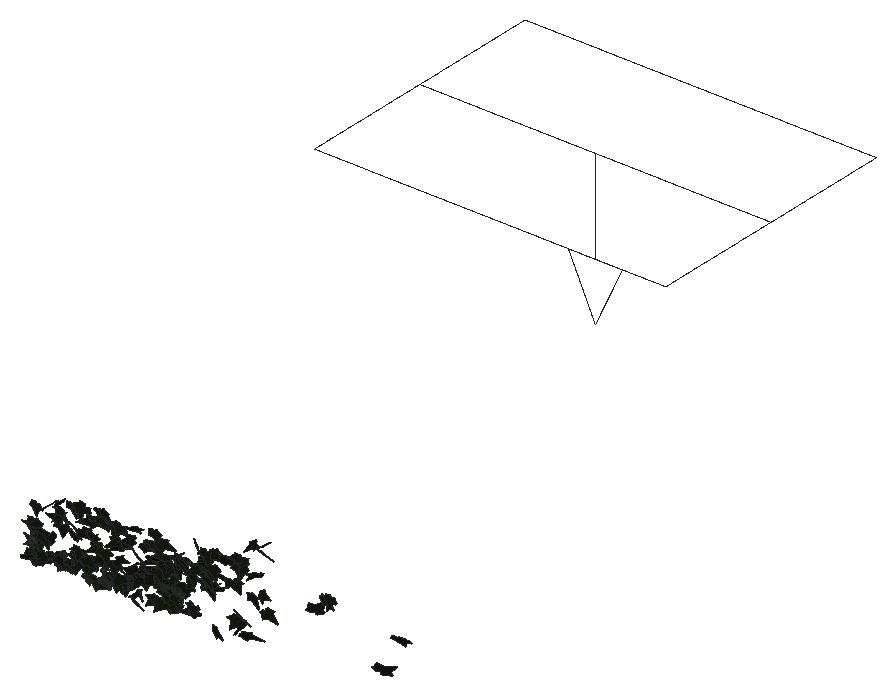
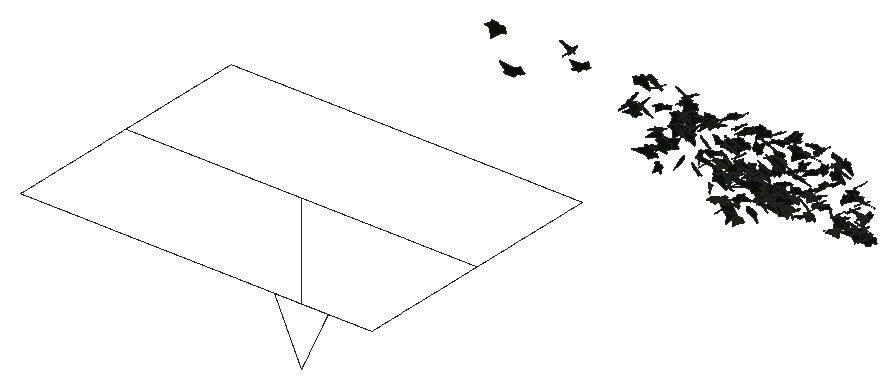
# SketchUp Ruby script. Lengths in millimetres.
U = 1.mm
M = Sketchup.active_model
def pt(a) = Geom::Point3d.new(a.map { |v| v * U })
def face(e, loops, mat)
  f = e.add_face(loops[0].map { |a| pt(a) })
  loops[1..].each { |l| e.add_face(l.map { |a| pt(a) }).erase! }
  f.material = f.back_material = mat if mat
  f
end
# faces: each face lists its corners as indices into pts; further lists are holes
def faces(e, pts, list, mat = nil) = list.each { |f| face(e, (f[0].is_a?(Array) ? f : [f]).map { |l| l.map { |i| pts[i] } }, mat) }
# xy, xz, yz: faces in a plane at the given z, y or x. An outline is a flat list of corners, or four numbers for a rectangle; further outlines are holes
def ring(l) = l.size == 4 ? [[l[0], l[1]], [l[2], l[1]], [l[2], l[3]], [l[0], l[3]]] : l.each_slice(2).to_a
def flat(e, list, mat, &to3) = list.each { |f| face(e, (f[0].is_a?(Array) ? f : [f]).map { |l| ring(l).map { |u, v| to3.(u, v) } }, mat) }
def xy(e, z, list, mat = nil) = flat(e, list, mat) { |x, y| [x, y, z] }
def xz(e, y, list, mat = nil) = flat(e, list, mat) { |x, z| [x, y, z] }
def yz(e, x, list, mat = nil) = flat(e, list, mat) { |y, z| [x, y, z] }
def lines(e, pts, list) = list.each { |a, b| e.add_line(pt(pts[a]), pt(pts[b])) }
# prism: a flat outline (further loops are holes) pulled along v
def prism(e, loops, v, mat = nil)
  f = face(e, loops, mat); d = Geom::Vector3d.new(v.map { |x| x * U })
  f.pushpull(f.normal.samedirection?(d) ? d.length : -d.length)
end
def box(e, o, s, mat = nil) = prism(e, [[o, [o[0] + s[0], o[1], o[2]], [o[0] + s[0], o[1] + s[1], o[2]], [o[0], o[1] + s[1], o[2]]]], [0, 0, s[2]], mat)
def at(x, y, z, deg = 0) = Geom::Transformation.translation(pt([x, y, z])) * Geom::Transformation.rotation(ORIGIN, Z_AXIS, deg.degrees)
def axes(o, x, y, z) = Geom::Transformation.new([*x, 0, *y, 0, *z, 0, *pt(o).to_a, 1])
def part(name) = M.definitions.add(name)
# library, detail: a bought-in or finely detailed component or shape, given as its bounding box
def library(name, o, s) = part(name).tap { |d| box(d.entities, o, s) }
def detail(e, o, s) = box(e.add_group.entities, o, s)
def put(e, d, t, mat = nil) = e.add_instance(d, t).tap { |i| i.material = mat if mat }
def group(e, t, mat = nil) = e.add_group.tap { |g| g.transformation = t; g.material = mat if mat }.entities
root = M.entities
M.materials.add("efeu1").color = [18, 25, 13]
M.materials.add("efeu2").color = [43, 57, 29]
c1 = part("ivyleaf_9")
p = [[39.1,54.8,31.7],[34.5,51.8,30.2],[-5.3,25.2,17.3],[-17.9,28.3,20.9],[-21.6,21.7,17],[-20.2,4.3,5.3],
  [-22.9,-0.3,2.5],[-17.1,-4,-0.6],[-2,-2.1,-1.2],[-0.7,-15.4,-10.1],[16.6,-22.3,-16.7],[21.1,-15.1,-12.5],
  [32.7,-10.7,-11],[46.1,-1.8,-6.6],[30.8,11.2,3.8]]
faces(c1.entities,p,[[0,1,2,3,4,5,6,7,8,9,10,11,12,13,14]],"efeu1")
c2 = part("ivyleaf_10")
p = [[0,12.8,-0.8],[-1.5,51.3,-10.9],[-4.9,51,-11.6],[-13.6,26.5,-7.3],[-13.2,15.9,-4.6],[-21.1,19.3,-7.2],
  [-29.5,16.3,-8.3],[-29.2,8.3,-6.2],[-19.7,-9.8,0.5],[-7.6,-13,4],[1,-12.2,5.8],[-0.4,51.1,-11.1],
  [-1.5,51.1,-10.9],[1,-12.4,5.9],[16.9,-12.4,3.5],[35.1,9.1,-5.1],[35,12.9,-6.1],[20.5,16.4,-4.9],
  [15.8,15,-3.8],[15.3,27.6,-7.1],[12.8,31.3,-7.8]]
faces(c2.entities,p,[[0,1,2,3,4,5,6,7,8,9,10],[11,12,0,13,14,15,16,17,18,19,20]],"efeu2")
c3 = part("Group257\#1")
p = [[0,0,0],[0,0,-959.4],[-272.7,0,-959.4],[1775.1,-1330.8,0],[-1775.1,-1330.8,0],[1775.1,1330.8,0],
  [1775.1,0,0],[-1775.1,1330.8,0],[272.7,0,-959.4],[-1775.1,0,0],[0,0,-1552.9]]
lines(c3.entities,p,[[0,1],[1,2],[3,4],[5,6],[7,5],[1,8],[9,0],[0,6],[8,10],[4,9],[6,3],[2,10],
  [9,7]])
c4 = part("Rectangle Light\#4")
put(c4.entities,c3,at(0,0,0))
put(root,c1,axes([7078.2,622.4,4794.7],[-1.245,-0.97894,0.63666],[-0.02381,-0.72384,-1.12583],[2.22236,-0.55617,0.34461]))
put(root,c2,axes([6934.9,593.1,4256.7],[-2.21181,-0.09357,-0.49205],[0.94502,-0.0521,-1.16284],[0.12508,-1.26095,0.08456]))
put(root,c1,axes([6281,585,4503.6],[2.52907,0.12258,-0.03253],[-0.06178,-0.00223,-1.33449],[-0.23333,1.32925,0.00076]))
put(root,c1,axes([6495.9,585.8,4670.1],[-1.29976,0.62888,0.92752],[-1.25598,0.65217,-0.92809],[-1.72371,-0.94941,-0.02314]))
put(root,c1,axes([6590.3,616.6,4820.6],[0.27311,-1.35729,0.14133],[0.01392,-0.14134,-1.36483],[2.59711,0.14349,-0.00755]))
put(root,c1,axes([6466.9,608.1,4738.9],[0.97787,-1.23155,-0.18048],[-0.14465,0.16385,-1.33441],[2.3645,0.51934,-0.00699]))
put(root,c1,axes([6744.1,595.8,4396.6],[0.64791,-0.91908,-0.92115],[-0.18486,0.93155,-0.96535],[2.46961,0.31086,0.16941]))
put(root,c1,axes([8009.6,616.5,4759.5],[-0.41068,-1.33295,-0.20263],[0.05642,0.20047,-1.3503],[2.5654,-0.21779,-0.00274]))
put(root,c1,axes([6918.3,615.8,4519.7],[-0.61056,-1.24261,-0.27622],[0.19455,0.25879,-1.28292],[2.41484,-0.33503,0.03352]))
put(root,c1,axes([6622.9,612.8,4311.1],[-1.63327,-0.68293,-0.61293],[0.92945,0.3706,-1.09668],[1.47861,-0.98732,0.01232]))
put(root,c1,axes([8044.7,595.2,4214.7],[1.52551,-0.81377,-0.91631],[-1.19527,0.66743,-1.14212],[2.00281,1.01816,0.01632]))
put(root,c1,axes([7850.7,609.5,4299.7],[-2.33926,0.27794,0.5582],[-1.02866,0.14045,-1.26005],[-0.59186,-1.34261,-0.01626]))
put(root,c1,axes([6390.5,631.9,4433.6],[-0.02071,-0.10759,1.41416],[-1.48401,-1.18083,-0.09584],[2.25466,-0.77821,-0.05009]))
put(root,c1,axes([7276.6,610.4,4576.3],[0.80844,-1.11543,0.79685],[-0.56507,0.73957,1.19352],[-2.54702,-0.51812,-0.01186]))
put(root,c1,axes([6402.3,601.3,4773.2],[-0.77594,1.19359,-0.3546],[0.06299,-0.3626,-1.25859],[-2.36893,-0.4006,0.08268]))
put(root,c1,axes([6634,625.9,4779],[0.47434,-1.23586,0.4161],[0.17935,-0.40546,-1.26069],[2.47534,0.2662,0.01161]))
put(root,c1,axes([7795.2,632,4600.8],[-0.27937,-1.24372,0.49099],[0.16104,-0.50159,-1.24527],[2.53972,-0.10501,0.13297]))
put(root,c1,axes([7504,623.9,4248.5],[-2.12366,-0.60101,-0.02105],[0.03428,0.01095,-1.2674],[1.14403,-1.11598,-0.0011]))
put(root,c1,axes([7229.7,595.6,4449.9],[-1.02657,0.98174,0.63763],[-0.921,0.45227,-1.10571],[-2.02867,-0.70212,0.17932]))
put(root,c1,axes([7208,605.4,4193.2],[2.05762,-0.66884,-0.30097],[-0.37912,0.24818,-1.26709],[1.3434,1.09446,0.1034]))
put(root,c1,axes([7500.5,595.2,4807.4],[0.76205,-0.5492,-1.21421],[0.12929,1.2746,-0.55411],[2.53298,0.10016,0.39358]))
put(root,c1,axes([7266.7,622.8,4393.1],[-2.10613,0.05032,-0.70148],[1.31881,-0.14542,-1.10359],[-0.22867,-1.30213,0.09614]))
put(root,c1,axes([6438.3,617,4296.1],[0.57814,-1.2113,-0.37192],[0.01779,0.38459,-1.24494],[2.41151,0.28756,0.09835]))
put(root,c1,axes([8560.5,606.4,4548.9],[0.61357,-1.05749,-0.93526],[-0.15117,0.94423,-1.09502],[2.68256,0.29508,0.15221]))
put(root,c1,axes([6579,614.5,4643.3],[1.97556,-0.82635,0.11102],[0.19213,-0.05141,-1.32659],[1.57517,1.04268,0.02257]))
put(root,c1,axes([7876.8,631.7,4680.3],[-2.31475,-0.23202,0.40606],[-0.5934,-0.441,-1.18586],[0.6634,-1.20401,0.3561]))
put(root,c1,axes([6132.4,628.2,4373.1],[1.08236,-1.03781,0.44412],[0.51604,-0.35715,-1.1818],[2.08552,0.62698,0.06193]))
put(root,c1,axes([8394.5,626.8,4630.2],[0.75629,-1.31613,-0.09347],[-0.06978,0.08657,-1.37477],[2.51019,0.39894,-0.01006]))
put(root,c1,axes([9717.4,611.8,4417.8],[-0.61084,-0.00029,1.42032],[2.65001,-0.28736,0.31459],[0.53334,1.42749,0.06362]))
put(root,c1,axes([7340.3,602,4731.9],[0.76226,-0.43282,-1.2469],[0.2578,1.30964,-0.41109],[2.49874,-0.00308,0.42279]))
put(root,c1,axes([7437.1,632,4745.2],[-0.19745,-1.33603,-0.1816],[-0.02194,0.18301,-1.33981],[2.56603,-0.10124,-0.02543]))
put(root,c1,axes([6701.1,633.6,4832.6],[-2.38193,-0.47755,-0.07895],[0.14095,0.02737,-1.33955],[0.91035,-1.25373,0.00083]))
put(root,c1,axes([6296.2,631.4,4255],[-2.275,0.08413,-0.39144],[0.70954,-0.21554,-1.18479],[-0.27787,-1.23921,0.1795]))
put(root,c2,axes([6902.4,629.9,4330.1],[1.32405,-1.01667,0.30384],[0.46548,-0.1999,-1.22888],[1.9651,0.73236,0.08637]))
put(root,c1,axes([6823.4,596.4,4598.7],[0.05355,0.16855,-1.30878],[-1.36437,1.101,0.12638],[2.1085,0.70815,0.11502]))
put(root,c1,axes([9893.2,607.7,4777.9],[2.48145,0.60112,-0.31814],[-0.54004,-0.14437,-1.43568],[-1.17637,1.3343,-0.01201]))
put(root,c1,axes([6765.5,631.8,4616.1],[0.9903,-1.19661,-0.04835],[-0.02932,0.04603,-1.30484],[2.27906,0.52054,0.00422]))
put(root,c1,axes([7404.4,636.3,4854.8],[0.27087,-1.32639,-0.08879],[0.03121,0.09104,-1.33375],[2.52984,0.14089,0.02596]))
put(root,c1,axes([7029,603.5,4586.3],[1.66456,0.16047,0.98959],[1.58884,0.61055,-0.83683],[-1.05642,1.1711,0.30068]))
put(root,c1,axes([6243.9,614.6,4501.1],[-1.2524,0.6636,0.93178],[-1.39566,0.5803,-0.93118],[-1.67093,-0.98209,0.07939]))
put(root,c1,axes([6832.8,629.3,4851.8],[1.55402,-1.05267,-0.13594],[-0.10535,0.12904,-1.33177],[2.01733,0.81765,0.03517]))
put(root,c1,axes([6865.1,631.8,4789.6],[0.44276,-1.24833,-0.40414],[0.05236,0.415,-1.26602],[2.49668,0.21267,0.09822]))
put(root,c1,axes([7935.2,642,4853.6],[-0.68157,-1.28837,-0.09768],[0.06076,0.0925,-1.33721],[2.45832,-0.35949,0.00597]))
put(root,c1,axes([8295.1,642,4849.2],[-1.93796,-0.15161,-0.85733],[1.65255,-0.27334,-0.98296],[-0.1212,-1.30275,0.30601]))
put(root,c1,axes([7341.2,626.5,4737.3],[1.50887,-1.05829,-0.35194],[-0.14928,0.37782,-1.31281],[2.11734,0.7808,0.15824]))
put(root,c1,axes([7041.2,643.4,4755.6],[-1.8811,-0.8944,-0.09871],[0.12954,0.0719,-1.33297],[1.70765,-0.9907,-0.00762]))
put(root,c1,axes([6466.8,604.9,4790.9],[-0.05691,1.1823,0.56334],[-0.16238,0.56053,-1.18094],[-2.48724,-0.06365,0.06421]))
put(root,c1,axes([6804.4,634.2,4731.5],[-2.20298,0.25758,0.63395],[-1.22704,0.00692,-1.17999],[-0.43641,-1.31973,0.11755]))
put(root,c1,axes([8260,648.8,4821.3],[-0.6842,-1.26365,0.20168],[0.17219,-0.23406,-1.30528],[2.42932,-0.33931,0.14932]))
put(root,c1,axes([7912.3,629,4586.3],[1.89664,-0.88618,-0.14908],[-0.20508,0.10317,-1.33357],[1.69794,1.00235,0.00546]))
put(root,c1,axes([9184,639.8,4874.8],[-2.14436,0.02339,-0.86278],[1.63757,-0.08103,-1.12584],[-0.12906,-1.41679,0.05015]))
put(root,c1,axes([7055.5,643.2,4323.3],[-2.13545,-0.49957,-0.40756],[0.76754,0.09442,-1.226],[0.95736,-1.19002,0.07382]))
put(root,c1,axes([6884.6,638.7,4854.6],[1.11664,-1.21149,-0.08961],[-0.09766,0.07471,-1.34602],[2.30994,0.5888,-0.01359]))
put(root,c1,axes([7659.6,642.3,4679.4],[0.70748,-1.3592,-0.17061],[-0.05053,0.1696,-1.40899],[2.60664,0.37219,0.01899]))
put(root,c1,axes([8439.3,633.8,4835.9],[0.03758,1.02003,-0.88375],[-0.27518,-0.87716,-1.01566],[-2.55382,0.10952,0.09644]))
put(root,c1,axes([7677.3,644.6,4692.6],[0.85234,-1.22621,0.06593],[0.04279,-0.06198,-1.30544],[2.33671,0.44841,-0.00014]))
put(root,c2,axes([6174.2,628.6,4359.7],[0.82399,1.17989,0.10803],[0.0123,0.11266,-1.25639],[-2.25492,0.43177,0.03262]))
put(root,c1,axes([7397.1,645.7,4413.4],[-2.38769,-0.09063,0.16456],[-0.31226,-0.01264,-1.25783],[0.17414,-1.26525,0.00078]))
put(root,c1,axes([6395.9,644.5,4293.5],[-0.44978,-1.14024,-0.51955],[0.80049,0.42584,-1.12592],[2.2464,-0.38005,0.29719]))
put(root,c1,axes([7189.3,634.2,4701],[-2.12457,0.62863,0.29212],[-0.46369,0.1626,-1.28096],[-1.23511,-1.14239,-0.02158]))
put(root,c1,axes([7775.9,663.1,4293],[-0.62335,-0.97207,0.78046],[-0.41583,-0.74969,-1.02545],[2.33583,-0.39288,0.02572]))
put(root,c1,axes([6107.8,638.5,4168.2],[2.06594,0.69081,0.17384],[-0.28626,-0.08744,1.28666],[1.32517,-1.09586,0.00692]))
put(root,c1,axes([7047.7,614.1,4484.9],[0.30462,0.06924,-1.32906],[-0.62488,1.29931,0.02815],[2.4546,0.32218,0.1721]))
put(root,c1,axes([7711.5,631.5,4703.7],[2.29619,-0.38811,0.45328],[0.9787,0.1575,-1.23388],[0.57619,1.27917,0.28945]))
put(root,c1,axes([8035.3,644.3,4871.9],[-2.25157,0.52033,-0.24498],[0.41055,-0.11794,-1.29225],[-1.01464,-1.20237,0.02074]))
put(root,c1,axes([8230.9,641.2,4409.7],[2.23134,-0.86353,0.02651],[0.0402,-0.01603,-1.4561],[1.64375,1.1726,-0.00038]))
put(root,c1,axes([9107.8,637.2,4855.4],[1.48503,-1.03601,-0.56814],[-0.45325,0.52897,-1.29167],[2.20261,0.80735,0.11725]))
put(root,c1,axes([7657.7,660.7,4691.5],[-1.3952,-1.09231,0.05257],[0.16275,-0.12035,-1.30825],[2.07492,-0.72504,0.13796]))
put(root,c1,axes([6290.2,656.6,4225.1],[-2.09746,-0.62143,0.03852],[-0.05541,-0.02679,-1.26517],[1.18368,-1.10242,0.00903]))
put(root,c1,axes([6466,658.9,4577.3],[-0.78808,-1.25309,-0.00492],[0.04773,-0.00311,-1.3195],[2.38442,-0.4141,0.02479]))
put(root,c1,axes([6453.7,651.2,4672.5],[-0.48978,0.84043,-0.97979],[0.35644,-0.9642,-0.87624],[-2.43077,-0.31073,0.06893]))
put(root,c1,axes([6268.4,654.4,4410.8],[0.03251,-1.28705,-0.21282],[0.03976,0.21308,-1.28695],[2.48246,0.01344,0.0234]))
put(root,c1,axes([6631.9,663.4,4404.1],[-1.07292,-1.14112,0.16814],[-0.08912,-0.16435,-1.27241],[2.19341,-0.56486,0.03055]))
put(root,c1,axes([6609.4,668.8,4330],[-1.26678,-0.96256,0.5463],[-0.25602,-0.5624,-1.15482],[2.09082,-0.65206,0.18958]))
put(root,c1,axes([6855.2,649.8,4506.7],[-2.40119,0.2257,0.22147],[-0.40424,0.07001,-1.28131],[-0.44585,-1.27904,-0.03105]))
put(root,c1,axes([7418.5,657.1,4497.4],[0.02606,-1.28329,-0.10753],[-0.00861,0.10748,-1.28336],[2.4509,0.01402,-0.00337]))
put(root,c2,axes([6713.6,640.3,4196.3],[-2.10863,0.56302,-0.13169],[0.23524,-0.04743,-1.24271],[-1.07502,-1.11473,-0.01363]))
put(root,c1,axes([7985.9,663.6,4658.7],[-0.18673,-1.2735,-0.30939],[-0.04251,-0.30858,1.27728],[-2.49387,0.10061,0.00139]))
put(root,c1,axes([7272,647.6,4383.7],[-2.24335,0.5102,-0.00308],[0.00394,-0.00296,-1.2844],[-0.97101,-1.17873,0.00189]))
put(root,c1,axes([7906.2,659.4,4608.7],[0.68906,-1.24979,0.15719],[0.08743,-0.15035,-1.30118],[2.39575,0.36495,0.00227]))
put(root,c1,axes([7410.3,669.5,4225.6],[-2.03702,-0.59375,0.4291],[-0.21936,-0.61377,-1.13677],[1.37686,-0.97621,0.45373]))
put(root,c1,axes([6189.6,668.7,4660.5],[-0.26425,-1.22781,0.42385],[-0.08049,-0.42177,-1.23562],[2.47077,-0.14506,0.00508]))
put(root,c2,axes([7024,664.1,4273.7],[0.14939,0.50649,-1.15391],[-1.57032,-0.85322,-0.43063],[-1.81281,0.78083,0.27794]))
put(root,c1,axes([9030.3,631,4712.2],[-1.02783,-0.1683,1.40716],[2.50069,0.50478,0.56465],[-1.01063,1.42019,-0.03394]))
put(root,c1,axes([6880.2,674,4189.3],[-1.09032,-0.82169,0.75071],[-0.61235,-0.68601,-0.9964],[2.02779,-0.64897,0.10276]))
put(root,c1,axes([6677.9,641.8,4609.2],[0.25944,-0.81519,-1.05838],[0.33002,1.06567,-0.79847],[2.52102,-0.05562,0.21344]))
put(root,c1,axes([6376.7,638.7,4253],[2.34574,0.18978,-0.27365],[-0.51935,-0.02575,-1.24695],[-0.36326,1.26228,0.0157]))
put(root,c1,axes([7393.5,635.7,4616.4],[2.23173,0.55782,-0.30408],[-0.5892,-0.0557,-1.29604],[-1.05587,1.21012,0.08051]))
put(root,c1,axes([6249.7,626.2,4187.1],[0.57436,0.83143,-1.063],[0.20048,1.07142,0.86792],[2.5606,-0.27038,0.17048]))
put(root,c1,axes([8189.6,651.9,4677.2],[-0.58219,-0.93967,-0.88934],[0.6008,0.83203,-0.9877],[2.38793,-0.43843,0.03168]))
put(root,c1,axes([6807.5,636,4742.1],[2.27969,0.60261,-0.08137],[-0.13149,-0.04373,-1.34084],[-1.14979,1.19978,-0.008]))
put(root,c1,axes([6980.3,663.5,4404.6],[-1.14177,-1.12921,-0.35348],[0.2354,0.3343,-1.27785],[2.2396,-0.61082,-0.0459]))
put(root,c1,axes([6983.4,665.5,4341.2],[-1.51958,0.57207,-0.85057],[0.79829,-0.80142,-0.93275],[-1.78008,-0.84776,0.3078]))
put(root,c1,axes([7197.7,656,4398.6],[1.04028,-1.11818,-0.39841],[-0.31082,0.36361,-1.24457],[2.23769,0.57034,0.01235]))
put(root,c2,axes([6703.2,651.9,4385.8],[-2.30465,0.34721,-0.14431],[0.20186,-0.15147,-1.25441],[-0.68656,-1.21006,0.11562]))
put(root,c1,axes([7939.5,640.3,4685.9],[0.10609,1.30094,-0.13778],[-0.29083,-0.13049,-1.2939],[-2.47276,0.07116,0.14627]))
put(root,c1,axes([8312,648.6,4889.6],[-1.35169,1.11665,-0.15151],[0.09572,-0.14751,-1.32287],[-2.14254,-0.71106,0.03648]))
put(root,c1,axes([7937.4,667.9,4522.9],[0.29813,-1.29976,0.00646],[0.00967,-0.00589,-1.30916],[2.47372,0.15667,0.00434]))
put(root,c1,axes([6616.4,678.1,4354.3],[-0.82908,-1.10953,0.50024],[-0.36815,-0.46145,-1.19194],[2.28692,-0.47653,-0.01053]))
put(root,c1,axes([8486.2,637.3,4664.6],[0.96675,-0.34775,-1.19551],[-1.17416,1.05121,-0.56791],[2.05823,0.76303,0.23755]))
put(root,c1,axes([7950,667.4,4532.3],[0.73825,0.03935,1.25108],[-2.37083,-0.11584,0.38988],[0.23276,-1.3047,0.00312]))
put(root,c1,axes([6165.2,673.8,4509.5],[-0.2332,-1.29694,0.07763],[0.20569,-0.08788,-1.29757],[2.46418,-0.1154,0.11566]))
put(root,c1,axes([7511.9,673,4556.1],[-1.76619,-0.8262,-0.34702],[0.54986,0.19704,-1.24175],[1.61442,-0.97098,0.04329]))
put(root,c1,axes([6782.9,668.2,4315.6],[-2.00137,0.42026,-0.5931],[1.03902,-0.23207,-1.13239],[-0.91343,-1.18479,0.01143]))
put(root,c1,axes([6798.1,659.9,4395.1],[-0.34626,-0.48036,-1.18869],[1.71379,0.80674,-0.46383],[1.73689,-0.89177,0.22069]))
put(root,c1,axes([7011.8,666,4613.4],[-2.30599,0.48754,-0.13641],[0.22239,-0.07495,-1.30579],[-0.9375,-1.21699,0.02578]))
put(root,c1,axes([7721,669.8,4689.1],[1.26229,-1.12809,0.03312],[0.06552,-0.01818,-1.30846],[2.14691,0.66382,0.02045]))
put(root,c1,axes([7169.2,645.1,4805.3],[2.04581,0.7792,0.06414],[0.08562,0.04723,-1.32759],[-1.48553,1.07581,0.01182]))
put(root,c1,axes([6200.7,684.7,4241.9],[-0.80215,-1.18848,0.26343],[0.05775,-0.28894,-1.25504],[2.3161,-0.40441,0.12253]))
put(root,c1,axes([6662.6,680,4281],[0.09629,-1.26886,0.1505],[-0.02528,-0.15114,-1.26973],[2.4317,0.04867,-0.01916]))
put(root,c1,axes([6249.4,669.6,4407.5],[-2.38988,0.27052,0.00943],[-0.01546,0.00705,-1.28452],[-0.51493,-1.25573,-0.00518]))
put(root,c1,axes([7494.4,659.5,4603.9],[-0.06084,1.19856,-0.54827],[-0.03632,-0.54879,-1.1986],[-2.50817,-0.02113,0.03066]))
put(root,c1,axes([7909.2,645.8,4793],[1.94943,0.80989,0.06334],[-0.02032,0.11535,-1.30218],[-1.54595,1.01974,0.09699]))
put(root,c1,axes([7177,649.9,4452.7],[-0.43721,1.28946,0.09858],[-0.0286,0.09746,-1.30977],[-2.4611,-0.2302,-0.00229]))
put(root,c1,axes([6992.3,675.9,4258.3],[0.38659,-1.26985,-0.15202],[-0.02636,0.15174,-1.28595],[2.43389,0.20334,0.01022]))
put(root,c2,axes([6480.5,671.7,4305.2],[1.30623,-1.06488,0.05864],[0.06032,-0.04933,-1.26689],[2.02885,0.68706,-0.00009]))
put(root,c1,axes([7690.4,676.8,4449.6],[-1.52573,-0.87771,-0.50482],[0.64965,0.37192,-1.18872],[1.81424,-0.87131,0.00112]))
put(root,c1,axes([7522.6,667.3,4623.7],[-2.11654,0.62478,0.25885],[-0.53874,0.0224,-1.27023],[-1.16891,-1.1416,0.11674]))
put(root,c2,axes([7439.1,666,4377.7],[-2.27583,0.34877,-0.24208],[0.37665,-0.18222,-1.24008],[-0.71486,-1.20636,0.11732]))
put(root,c1,axes([7182.6,684,4385.1],[-0.25054,-1.28628,0.02232],[0.08585,-0.02704,-1.29213],[2.44692,-0.13075,0.04762]))
put(root,c1,axes([7398.7,691.8,4380.4],[-0.64751,-0.28023,1.19531],[-0.0287,-1.23931,-0.29484],[2.33641,-0.09289,0.32764]))
put(root,c1,axes([7580.6,662.2,4462.1],[-1.54378,0.99047,0.0013],[0.05987,0.02744,-1.27955],[-1.88411,-0.81068,-0.04172]))
put(root,c1,axes([7775.6,645,4496],[-0.19402,0.85981,0.97278],[-0.49334,0.94265,-0.86035],[-2.42117,-0.26097,0.09735]))
put(root,c2,axes([6162.9,658.4,4314.2],[-1.01238,1.07296,0.40355],[-0.6291,0.28241,-1.1866],[-2.08904,-0.60502,0.16177]))
put(root,c1,axes([6556.1,653.4,4536.7],[1.79131,-0.29583,-0.85126],[-1.12853,0.72361,-0.90709],[1.29158,1.04255,0.38804]))
put(root,c1,axes([6132.9,689.4,4197.5],[-0.37813,-1.24298,0.18906],[-0.01036,-0.19056,-1.25852],[2.39282,-0.19725,0.02443]))
put(root,c1,axes([7446.8,686.9,4363.1],[0.91308,0.42525,1.37572],[-2.2224,-0.73357,0.63398],[1.60352,-1.25883,0.0953]))
put(root,c1,axes([6784.5,688.9,4187.4],[-1.18504,-1.11776,-0.06517],[0.31023,-0.01672,-1.27063],[2.10823,-0.62583,0.15034]))
put(root,c1,axes([7020.9,657.1,4596.5],[-0.03495,1.30968,-0.03439],[-0.41757,-0.03698,-1.29123],[-2.45823,-0.01234,0.21983]))
put(root,c1,axes([6981.4,689.9,4235.9],[-0.8419,-1.16717,0.01331],[0.24528,-0.06299,-1.23999],[2.20793,-0.43805,0.14283]))
put(root,c1,axes([7600.6,682.3,4588.5],[-1.2913,-0.09135,-1.09196],[2.08071,0.03031,-0.68184],[0.14085,-1.28522,0.06154]))
put(root,c1,axes([7585.8,690.4,4291.8],[-0.17226,-1.27467,0.05842],[-0.06901,-0.05597,-1.27747],[2.42751,-0.09204,-0.03217]))
put(root,c1,axes([8298.7,661.8,4227.6],[0.65552,0.34846,-1.27601],[1.60124,0.95973,0.48919],[1.94253,-0.9087,0.02736]))
put(root,c1,axes([7940,669.5,4532],[0.06907,1.18323,-0.56362],[-0.43804,-0.54932,-1.16802],[-2.45558,0.13127,0.1925]))
put(root,c1,axes([7843.8,655.1,4706.9],[1.44105,1.03684,0.2149],[0.27956,0.15879,-1.28364],[-1.99577,0.77089,-0.02464]))
put(root,c1,axes([6950.7,686,4243.2],[1.35472,-1.1333,0.21021],[0.24513,-0.16731,-1.33816],[2.17996,0.7231,0.01984]))
put(root,c1,axes([6158.2,688.5,4293.8],[-0.31745,-1.26165,-0.18275],[-0.00417,0.18459,-1.27236],[2.42623,-0.16476,-0.0261]))
put(root,c1,axes([6181.6,689.7,4318.9],[0.2848,-1.27223,-0.00027],[-0.01483,-0.00065,-1.28098],[2.42127,0.14964,-0.00781]))
put(root,c1,axes([7533.8,673.8,4570.6],[-1.87448,0.8125,0.05806],[-0.0912,0.03314,-1.27678],[-1.5476,-0.98606,0.00492]))
put(root,c1,axes([7351.7,687.6,4406.6],[-2.37855,0.19654,-0.06045],[0.06067,-0.18269,-1.25292],[-0.38662,-1.23782,0.17532]))
put(root,c1,axes([7993.5,663.8,4556.6],[-0.25996,1.30686,-0.01214],[0.0004,-0.01218,-1.31397],[-2.48731,-0.13659,0.00106]))
put(root,c1,axes([7213.2,694.6,4339.1],[0.52168,-1.19673,0.34469],[0.37669,-0.30659,-1.22186],[2.34008,0.31614,0.11984]))
put(root,c1,axes([7028.9,699.1,4267.1],[-0.07516,-1.15836,0.48367],[0.49721,-0.4809,-1.13039],[2.33674,0.06507,0.25608]))
put(root,c1,axes([6353.6,691.3,4234.7],[0.48532,-1.25601,0.00718],[0.00014,-0.00731,-1.28163],[2.39047,0.255,-0.00138]))
put(root,c1,axes([7984.8,668.4,4673.1],[-0.55268,1.26792,-0.1074],[-0.26128,-0.14074,-1.29028],[-2.40761,-0.27579,0.16468]))
put(root,c1,axes([8216.3,694.9,4319.4],[-2.26028,-0.62225,-0.08711],[0.1711,0.01607,-1.34048],[1.18352,-1.1907,0.02743]))
put(root,c1,axes([7477.8,694.7,4321.1],[-0.83974,-1.16685,-0.26044],[0.17089,0.24448,-1.24748],[2.26897,-0.45026,-0.00243]))
put(root,c1,axes([7419.8,684.9,4445.3],[-1.7095,0.87982,-0.14322],[-0.22618,-0.3197,-1.21864],[-1.68137,-0.85153,0.30955]))
put(root,c1,axes([7522,697.9,4398.5],[1.03536,-0.71336,0.89818],[1.03286,-0.71568,-0.89712],[1.92316,0.76842,-0.00173]))
put(root,c1,axes([7263.7,684.4,4455.7],[1.77942,-0.88647,-0.04828],[0.25279,0.209,-1.2653],[1.67061,0.91258,0.24288]))
put(root,c1,axes([7287.4,704.3,4380.6],[-0.6798,-1.20418,0.11684],[0.01691,-0.12443,-1.25528],[2.3025,-0.35461,0.04372]))
put(root,c1,axes([7588.1,698,4284.8],[-2.39311,-0.19818,0.02701],[-0.05144,-0.00198,-1.27293],[0.37718,-1.2577,-0.00225]))
put(root,c2,axes([7204.4,700.6,4203.2],[0.73016,-0.89436,0.77072],[1.45364,-0.42994,-0.87912],[1.71342,0.74588,0.41739]))
put(root,c1,axes([7613.8,679.1,4209],[-1.24004,0.79803,0.75259],[-1.30454,0.38719,-1.004],[-1.62988,-0.91706,0.23101]))
put(root,c1,axes([6943.4,681.6,4282.3],[1.19669,0.88608,-0.70008],[-0.7394,-0.58264,-1.08637],[-2.01803,0.73892,-0.0171]))
put(root,c1,axes([7454.1,698.5,4225.3],[0.52013,-1.23369,-0.12422],[-0.04053,0.12251,-1.26359],[2.35949,0.27406,0.00568]))
put(root,c1,axes([6131.4,681.2,4229.5],[1.62246,-0.69042,-0.61294],[-0.63608,0.54691,-1.08088],[1.63794,0.89628,0.1874]))
put(root,c1,axes([6178.9,696.5,4327.6],[-2.2202,0.47717,-0.12141],[0.07547,-0.22015,-1.2463],[-0.93405,-1.15201,0.18788]))
put(root,c1,axes([8019.7,669,4540.2],[1.29652,1.08107,0.28056],[0.17807,0.27224,-1.27618],[-2.11817,0.6846,0.06445]))
put(root,c1,axes([7254.2,673,4431.2],[1.80674,0.85928,0.09773],[0.12357,0.07389,-1.28041],[-1.64128,0.95147,0.01118]))
put(root,c1,axes([7088.8,670.2,4584],[-0.39516,1.04748,0.75387],[-0.38864,0.72728,-1.06677],[-2.42524,-0.28722,0.04812]))
put(root,c1,axes([7430,705.1,4347.8],[1.02465,-1.1048,0.28439],[0.26577,-0.24828,-1.22889],[2.15487,0.55596,0.01634]))
put(root,c2,axes([6891.7,700.1,4230.7],[-1.9197,-0.76342,0.01216],[0.453,-0.33355,-1.19686],[1.38072,-0.952,0.40959]))
put(root,c2,axes([7182.5,690.7,4367.8],[-2.2104,0.49647,-0.12463],[0.20853,-0.06074,-1.26301],[-0.95161,-1.1665,0.01272]))
put(root,c1,axes([6408,696.9,4209],[0.76681,-1.12234,-0.44563],[0.51437,0.54167,-1.11988],[2.23996,0.25983,0.40972]))
put(root,c2,axes([6141.4,696.2,4410.7],[-2.1635,0.53844,0.18506],[-0.62478,-0.28222,-1.1954],[-0.88533,-1.11662,0.39136]))
put(root,c1,axes([7987,685.6,4660.9],[2.45895,0.06514,-0.12699],[-0.24093,-0.01104,-1.29364],[-0.12544,1.29818,-0.00462]))
put(root,c1,axes([7054.3,693.8,4334.6],[2.0245,-0.68486,0.17281],[0.53916,0.12751,-1.23852],[1.23142,1.07011,0.25817]))
put(root,c1,axes([7299.3,682.7,4342.6],[-0.83527,0.61683,1.00301],[-1.17946,0.78917,-0.75649],[-1.90553,-0.75885,0.02858]))
put(root,c1,axes([7289.1,692,4425.3],[-1.14003,0.21651,1.10848],[1.97854,-0.3847,0.63692],[0.84012,1.19981,0.0042]))
put(root,c2,axes([7099.5,699.3,4307],[-1.26303,-1.0746,0.04055],[-0.0668,-0.02598,-1.2629],[2.04554,-0.66436,-0.0162]))
put(root,c2,axes([6950.9,706.5,4235.2],[0.15843,-1.24369,0.17658],[-0.00061,-0.17699,-1.24641],[2.39072,0.08237,-0.01202]))
put(root,c2,axes([6904.8,700.2,4204.8],[-0.93926,-1.16352,-0.08017],[0.09796,0.06523,-1.26367],[2.2175,-0.49571,0.02187]))
put(root,c2,axes([6427.1,706.5,4185.1],[1.7552,0.70496,-0.47769],[-0.82228,-0.21943,-1.15795],[-1.39661,1.01516,0.08143]))
put(root,c2,axes([6862.3,707.2,4205.5],[1.05558,-1.12895,0.04152],[0.05206,-0.03283,-1.2578],[2.14945,0.55522,0.01007]))
put(root,c2,axes([7127.4,706.6,4306.8],[-0.57537,-1.21917,0.07984],[-0.01215,-0.08067,-1.25603],[2.32527,-0.3021,0.01319]))
put(root,c2,axes([7239.3,698.8,4360.5],[2.0368,-0.45992,-0.50399],[-0.65512,0.44551,-1.13749],[1.12118,1.09583,0.25092]))
put(root,c1,axes([7039.7,714.9,4214.7],[-0.99893,-1.07341,-0.35701],[0.33375,0.3116,-1.1947],[2.12692,-0.55303,0.0198]))
put(root,c1,axes([7600.8,689.6,4312.5],[-0.22285,1.27595,-0.00124],[-0.00036,-0.00126,-1.28132],[-2.4284,-0.11709,0.0003]))
put(root,c1,axes([7194,697,4191],[-1.22451,1.06538,-0.06382],[0.07045,-0.0522,-1.24458],[-2.03004,-0.64444,-0.0047]))
put(root,c1,axes([7238.8,694.3,4309.6],[0.12654,1.23552,-0.18182],[0.05809,-0.18363,-1.23666],[-2.37606,0.06131,-0.03992]))
put(root,c2,axes([7106.9,700.2,4265.9],[-1.75913,0.82505,0.09608],[-0.13035,0.06756,-1.23896],[-1.57547,-0.92682,-0.00478]))
put(root,c1,axes([6383,679.5,4270.9],[0.87421,0.78995,0.89487],[0.5071,0.86679,-0.90193],[-2.21444,0.51034,0.14673]))
put(root,c2,axes([7003.3,718.1,4209.6],[0.78504,-1.15487,0.20059],[0.17576,-0.17997,-1.22604],[2.22391,0.42189,0.02609]))
put(root,c2,axes([7051,715.6,4240],[2.02381,-0.50755,0.41179],[0.83853,-0.02421,-1.16758],[0.9188,1.14006,0.15854]))
put(root,c2,axes([7570.5,713.6,4401.5],[2.32584,-0.2873,0.16471],[0.37939,0.13529,-1.24301],[0.50331,1.22568,0.17581]))
put(root,c1,axes([7102.1,699.6,4294.7],[2.00467,-0.1652,-0.6635],[-1.08151,0.46619,-1.01821],[0.72371,1.15428,0.31627]))
put(root,c1,axes([6922,709.5,4189.3],[1.1725,-0.00289,1.09485],[2.05924,0.19367,-0.60832],[-0.31857,1.24126,0.09746]))
put(root,c2,axes([7501.2,742.1,4316.6],[2.00558,-0.41487,-0.54309],[-0.82544,0.36539,-1.12068],[1.00521,1.12779,0.1633]))
put(root,c1,axes([7165.6,740.5,4338.5],[1.86915,-0.15036,1.11304],[2.08782,-0.18875,-0.99346],[0.45853,1.47234,-0.01369]))
put(root,c1,axes([8162.6,740.4,4186.2],[-0.24676,0.40737,-1.26995],[-1.35138,1.05899,0.41219],[2.14863,0.71284,0.1134]))
put(root,c2,axes([7466.3,911,4208.6],[1.41712,1.00185,-0.18775],[-0.24846,-0.13686,-1.24804],[-1.92394,0.75561,0.02288]))
put(root,c1,axes([8007.6,983.8,4675.9],[-1.34927,-1.14555,0.14185],[0.16175,-0.21782,-1.3343],[2.19091,-0.68941,0.18587]))
put(root,c1,axes([7870.5,981.7,4582.4],[1.15276,-0.32306,1.15179],[-1.87787,0.59501,0.68576],[-1.28721,-1.15735,0.03105]))
put(root,c1,axes([7158.8,1001.2,4362.7],[-0.09587,-0.10713,-1.26314],[0.11122,-1.26299,0.10479],[-2.41008,-0.05402,0.05508]))
put(root,c1,axes([8134.7,992.3,4838.5],[-1.93388,0.67049,-0.50136],[0.65578,-0.38364,-1.21141],[-1.45217,-1.06615,0.12061]))
put(root,c1,axes([7594.6,1007.2,4487.2],[-1.74778,0.42729,-0.85127],[1.2852,-0.54188,-1.00047],[-1.27845,-1.12888,0.15803]))
put(root,c1,axes([7358.5,987.1,4476.6],[-0.07144,1.22839,-0.38138],[-0.07363,-0.38245,-1.22802],[-2.44686,-0.02435,0.04809]))
put(root,c1,axes([7241.3,1012.7,4293],[-2.28353,-0.29103,-0.13396],[0.36193,-0.22908,-1.20566],[0.49071,-1.18536,0.26589]))
put(root,c2,axes([7129.7,995,4360.6],[-0.80032,1.18964,-0.00915],[0.00692,-0.00842,-1.26177],[-2.26418,-0.42053,-0.00062]))
put(root,c2,axes([7424.1,1026.1,4360.7],[-0.18854,0.22167,-1.23551],[-0.06498,-1.23937,-0.21963],[-2.38808,0.01622,0.10352]))
put(root,c1,axes([8159.7,1005.5,4792.6],[2.0815,-0.66247,0.31522],[0.56323,-0.11939,-1.27771],[1.27762,1.13192,0.04972]))
put(root,c2,axes([7310.3,1010.7,4308.9],[1.10121,1.01382,-0.44515],[-0.41876,-0.38697,-1.16731],[-2.06528,0.61903,-0.00067]))
put(root,c1,axes([7033.2,991.8,4287.2],[-0.66486,1.18854,0.11043],[-0.02986,0.11048,-1.23871],[-2.27157,-0.34932,-0.01604]))
put(root,c1,axes([7541.1,993,4631.2],[1.0285,-0.09807,-1.18016],[-1.96333,0.59806,-0.52208],[1.1068,1.15201,0.17056]))
put(root,c1,axes([7258.9,1020.6,4263.3],[-0.54518,0.88755,-0.82327],[-0.02927,-0.8486,-0.90951],[-2.3038,-0.19925,0.20638]))
put(root,c1,axes([7212.6,1008.5,4203.4],[1.92815,-0.16758,-0.77942],[-1.38268,0.32493,-1.01419],[0.62479,1.23625,0.16091]))
put(root,c1,axes([7284.7,1027.3,4229.8],[0.97822,-1.05442,-0.41332],[-0.27649,0.38876,-1.17242],[2.13763,0.53281,0.0375]))
put(root,c2,axes([7266,1022.3,4302.2],[1.07732,1.07405,0.2793],[0.16542,0.26967,-1.21315],[-2.10562,0.57071,0.0476]))
put(root,c1,axes([7867.7,1016.5,4611.6],[2.41123,0.10204,-0.21876],[-0.4322,0.10754,-1.26501],[-0.15577,1.28118,0.1236]))
put(root,c1,axes([8203.6,1013.2,4844.4],[0.44456,1.2735,0.24605],[0.15577,0.23503,-1.29421],[-2.46363,0.24467,-0.03743]))
put(root,c2,axes([7130.6,1038.4,4194.5],[-1.09338,-0.92797,-0.57674],[0.77387,0.42321,-1.08598],[1.93006,-0.69539,0.10871]))
put(root,c4,at(7805.4,5705.2,6197.3))
